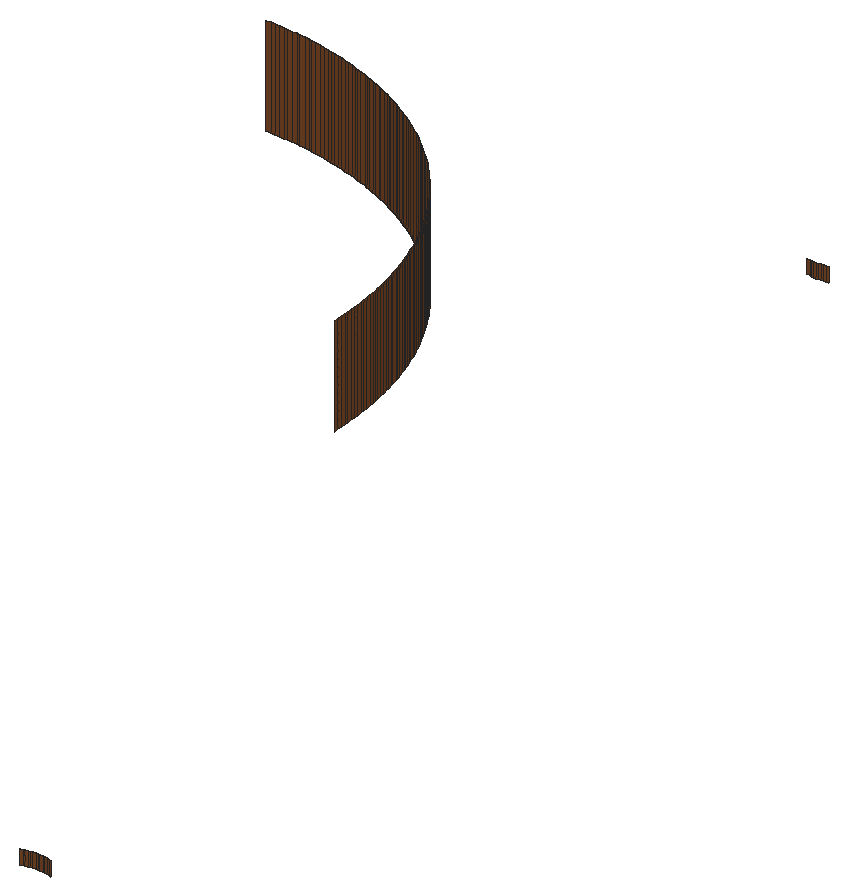
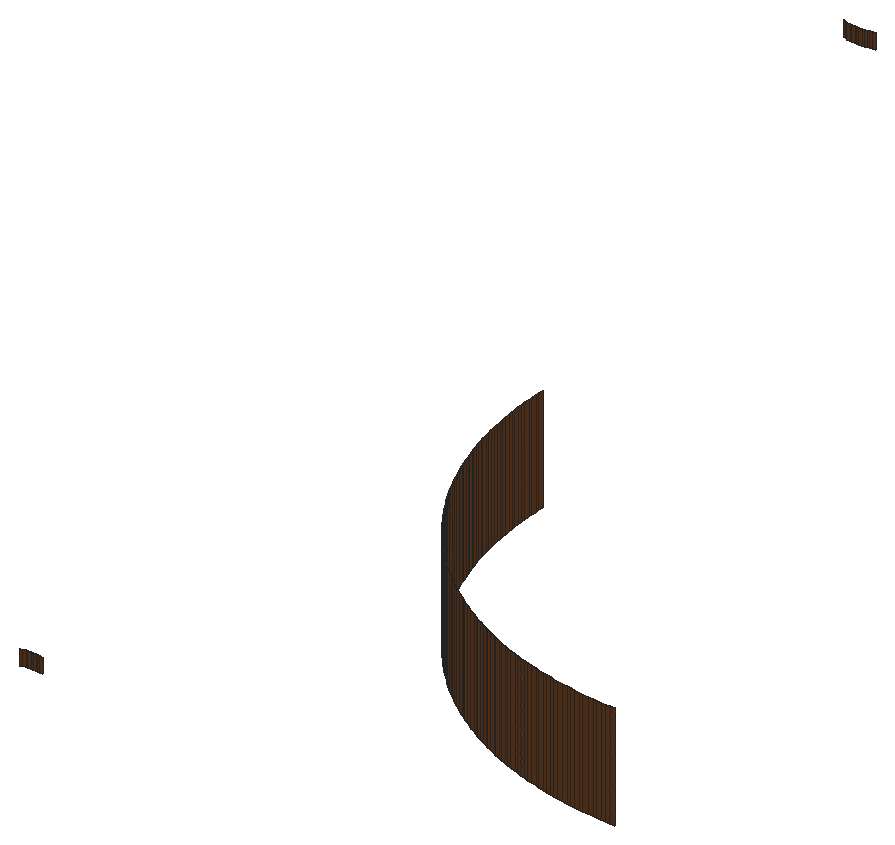
# SketchUp Ruby script. Lengths in inches.
U = 1.inch
M = Sketchup.active_model
def pt(a) = Geom::Point3d.new(a.map { |v| v * U })
def face(e, loops, mat)
  f = e.add_face(loops[0].map { |a| pt(a) })
  loops[1..].each { |l| e.add_face(l.map { |a| pt(a) }).erase! }
  f.material = f.back_material = mat if mat
  f
end
# faces: each face lists its corners as indices into pts; further lists are holes
def faces(e, pts, list, mat = nil) = list.each { |f| face(e, (f[0].is_a?(Array) ? f : [f]).map { |l| l.map { |i| pts[i] } }, mat) }
# xy, xz, yz: faces in a plane at the given z, y or x. An outline is a flat list of corners, or four numbers for a rectangle; further outlines are holes
def ring(l) = l.size == 4 ? [[l[0], l[1]], [l[2], l[1]], [l[2], l[3]], [l[0], l[3]]] : l.each_slice(2).to_a
def flat(e, list, mat, &to3) = list.each { |f| face(e, (f[0].is_a?(Array) ? f : [f]).map { |l| ring(l).map { |u, v| to3.(u, v) } }, mat) }
def xy(e, z, list, mat = nil) = flat(e, list, mat) { |x, y| [x, y, z] }
def xz(e, y, list, mat = nil) = flat(e, list, mat) { |x, z| [x, y, z] }
def yz(e, x, list, mat = nil) = flat(e, list, mat) { |y, z| [x, y, z] }
def lines(e, pts, list) = list.each { |a, b| e.add_line(pt(pts[a]), pt(pts[b])) }
# prism: a flat outline (further loops are holes) pulled along v
def prism(e, loops, v, mat = nil)
  f = face(e, loops, mat); d = Geom::Vector3d.new(v.map { |x| x * U })
  f.pushpull(f.normal.samedirection?(d) ? d.length : -d.length)
end
def box(e, o, s, mat = nil) = prism(e, [[o, [o[0] + s[0], o[1], o[2]], [o[0] + s[0], o[1] + s[1], o[2]], [o[0], o[1] + s[1], o[2]]]], [0, 0, s[2]], mat)
def at(x, y, z, deg = 0) = Geom::Transformation.translation(pt([x, y, z])) * Geom::Transformation.rotation(ORIGIN, Z_AXIS, deg.degrees)
def axes(o, x, y, z) = Geom::Transformation.new([*x, 0, *y, 0, *z, 0, *pt(o).to_a, 1])
def part(name) = M.definitions.add(name)
# library, detail: a bought-in or finely detailed component or shape, given as its bounding box
def library(name, o, s) = part(name).tap { |d| box(d.entities, o, s) }
def detail(e, o, s) = box(e.add_group.entities, o, s)
def put(e, d, t, mat = nil) = e.add_instance(d, t).tap { |i| i.material = mat if mat }
def group(e, t, mat = nil) = e.add_group.tap { |g| g.transformation = t; g.material = mat if mat }.entities
root = M.entities
M.materials.add("[Wood Veneer 01]3").color = [120, 70, 37]
xz(root,128.66,[[147.1,118,147.18,118.5]],"[Wood Veneer 01]3")
xz(root,128.67,[[146.93,118,147.01,118.5]],"[Wood Veneer 01]3")
xz(root,165,[[126,118,126.16,121.5],[126.16,118,126.3125,121.5]],"[Wood Veneer 01]3")
xz(root,168,[[142.9,118,142.99,118.5],[142.99,118,143.07,118.5]],"[Wood Veneer 01]3")
xz(root,168.01,[[143.15,118,143.24,118.5]],"[Wood Veneer 01]3")
yz(root,138,[[153,118,153.16,121.5],[153.16,118,153.3125,121.5]],"[Wood Veneer 01]3")
p = [[146.44,128.59,118],[146.52,128.61,118],[146.52,128.61,118.5],[146.44,128.59,118.5],[146.6,128.625,118],[146.6,128.625,118.5],
  [146.68,128.64,118],[146.68,128.64,118.5],[146.76,128.65,118],[146.76,128.65,118.5],[147.18,128.66,118],[147.26,128.65,118],
  [147.26,128.65,118.5],[147.18,128.66,118.5],[147.35,128.64,118],[147.43,128.62,118],[147.43,128.62,118.5],[147.35,128.64,118.5],
  [147.51,128.6,118],[147.51,128.6,118.5],[146.85,128.66,118],[146.85,128.66,118.5],[146.93,128.67,118],[146.93,128.67,118.5],
  [147.01,128.67,118],[147.1,128.66,118],[147.1,128.66,118.5],[147.01,128.67,118.5],[138,153.3125,118],[138,153.3125,121],
  [138,153.3125,121.5],[137.99,153.47,121.5],[137.99,153.47,121],[137.99,153.47,118],[137.98,153.63,121.5],[137.98,153.63,121],
  [137.98,153.63,118],[137.97,153.78,121.5],[137.97,153.78,121],[137.97,153.78,118],[137.96,153.94,121.5],[137.96,153.94,121],
  [137.96,153.94,118],[137.95,154.1,121.5],[137.95,154.1,121],[137.95,154.1,118],[137.93,154.25,121.5],[137.93,154.25,121],
  [137.93,154.25,118],[137.92,154.41,121.5],[137.92,154.41,121],[137.92,154.41,118],[137.9,154.57,121.5],[137.9,154.57,121],
  [137.9,154.57,118],[137.875,154.72,121.5],[137.875,154.72,121],[137.875,154.72,118],[137.85,154.88,121.5],[137.85,154.88,121],
  [137.85,154.88,118],[137.83,155.03,121.5],[137.83,155.03,121],[137.83,155.03,118],[137.8,155.1875,121.5],[137.8,155.1875,121],
  [137.8,155.1875,118],[137.77,155.34,121.5],[137.77,155.34,121],[137.77,155.34,118],[137.74,155.49,121.5],[137.74,155.49,121],
  [137.74,155.49,118],[137.7,155.65,121.5],[137.7,155.65,121],[137.7,155.65,118],[137.67,155.8,121.5],[137.67,155.8,121],
  [137.67,155.8,118],[137.63,155.95,121.5],[137.63,155.95,121],[137.63,155.95,118],[137.59,156.11,121.5],[137.59,156.11,121],
  [137.59,156.11,118],[137.55,156.26,121.5],[137.55,156.26,121],[137.55,156.26,118],[137.51,156.41,121.5],[137.51,156.41,121],
  [137.51,156.41,118],[137.46,156.56,121.5],[137.46,156.56,121],[137.46,156.56,118],[137.41,156.71,121.5],[137.41,156.71,121],
  [137.41,156.71,118],[137.36,156.86,121.5],[137.36,156.86,121],[137.36,156.86,118],[137.3125,157.01,121.5],[137.3125,157.01,121],
  [137.3125,157.01,118],[137.26,157.15,121.5],[137.26,157.15,121],[137.26,157.15,118],[137.2,157.3,121.5],[137.2,157.3,121],
  [137.2,157.3,118],[137.15,157.45,121.5],[137.15,157.45,121],[137.15,157.45,118],[137.09,157.59,121.5],[137.09,157.59,121],
  [137.09,157.59,118],[137.03,157.74,121.5],[137.03,157.74,121],[137.03,157.74,118],[136.96,157.88,121.5],[136.96,157.88,121],
  [136.96,157.88,118],[136.9,158.02,121.5],[136.9,158.02,121],[136.9,158.02,118],[136.83,158.17,121.5],[136.83,158.17,121],
  [136.83,158.17,118],[136.76,158.31,121.5],[136.76,158.31,121],[136.76,158.31,118],[136.69,158.45,121.5],[136.69,158.45,121],
  [136.69,158.45,118],[136.62,158.59,121.5],[136.62,158.59,121],[136.62,158.59,118],[136.55,158.73,121.5],[136.55,158.73,121],
  [136.55,158.73,118],[136.47,158.86,121.5],[136.47,158.86,121],[136.47,158.86,118],[136.39,159,121.5],[136.39,159,121],
  [136.39,159,118],[136.3125,159.14,121.5],[136.3125,159.14,121],[136.3125,159.14,118],[136.23,159.27,121.5],[136.23,159.27,121],
  [136.23,159.27,118],[136.15,159.4,121.5],[136.15,159.4,121],[136.15,159.4,118],[136.0625,159.54,121.5],[136.0625,159.54,121],
  [136.0625,159.54,118],[135.98,159.67,121.5],[135.98,159.67,121],[135.98,159.67,118],[135.89,159.8,121.5],[135.89,159.8,121],
  [135.89,159.8,118],[135.8,159.93,121.5],[135.8,159.93,121],[135.8,159.93,118],[135.71,160.05,121.5],[135.71,160.05,121],
  [135.71,160.05,118],[135.62,160.18,121.5],[135.62,160.18,121],[135.62,160.18,118],[135.52,160.31,121.5],[135.52,160.31,121],
  [135.52,160.31,118],[135.42,160.43,121.5],[135.42,160.43,121],[135.42,160.43,118],[135.33,160.55,121.5],[135.33,160.55,121],
  [135.33,160.55,118],[135.23,160.67,121.5],[135.23,160.67,121],[135.23,160.67,118],[135.125,160.79,121.5],[135.125,160.79,121],
  [135.125,160.79,118],[135.02,160.91,121.5],[135.02,160.91,121],[135.02,160.91,118],[134.92,161.03,121.5],[134.92,161.03,121],
  [134.92,161.03,118],[134.8125,161.15,121.5],[134.8125,161.15,121],[134.8125,161.15,118],[134.7,161.26,121.5],[134.7,161.26,121],
  [134.7,161.26,118],[134.6,161.375,121.5],[134.6,161.375,121],[134.6,161.375,118],[134.49,161.49,121.5],[134.49,161.49,121],
  [134.49,161.49,118],[134.375,161.6,121.5],[134.375,161.6,121],[134.375,161.6,118],[134.26,161.7,121.5],[134.26,161.7,121],
  [134.26,161.7,118],[134.15,161.8125,121.5],[134.15,161.8125,121],[134.15,161.8125,118],[134.03,161.92,121.5],[134.03,161.92,121],
  [134.03,161.92,118],[133.91,162.02,121.5],[133.91,162.02,121],[133.91,162.02,118],[133.79,162.125,121.5],[133.79,162.125,121],
  [133.79,162.125,118],[133.67,162.23,121.5],[133.67,162.23,121],[133.67,162.23,118],[133.55,162.33,121.5],[133.55,162.33,121],
  [133.55,162.33,118],[133.43,162.42,121.5],[133.43,162.42,121],[133.43,162.42,118],[133.31,162.52,121.5],[133.31,162.52,121],
  [133.31,162.52,118],[133.18,162.62,121.5],[133.18,162.62,121],[133.18,162.62,118],[133.05,162.71,121.5],[133.05,162.71,121],
  [133.05,162.71,118],[132.93,162.8,121.5],[132.93,162.8,121],[132.93,162.8,118],[132.8,162.89,121.5],[132.8,162.89,121],
  [132.8,162.89,118],[132.67,162.98,121.5],[132.67,162.98,121],[132.67,162.98,118],[132.54,163.0625,121.5],[132.54,163.0625,121],
  [132.54,163.0625,118],[132.4,163.15,118],[132.4,163.15,121],[132.4,163.15,121.5],[132.27,163.23,121.5],[132.27,163.23,121],
  [132.27,163.23,118],[132.14,163.3125,121.5],[132.14,163.3125,121],[132.14,163.3125,118],[132,163.39,121.5],[132,163.39,121],
  [132,163.39,118],[131.86,163.47,121.5],[131.86,163.47,121],[131.86,163.47,118],[131.73,163.55,118],[131.73,163.55,121],
  [131.73,163.55,121.5],[131.59,163.62,121.5],[131.59,163.62,121],[131.59,163.62,118],[131.45,163.69,121.5],[131.45,163.69,121],
  [131.45,163.69,118],[131.31,163.76,121.5],[131.31,163.76,121],[131.31,163.76,118],[131.17,163.83,118],[131.17,163.83,121],
  [131.17,163.83,121.5],[131.02,163.9,121.5],[131.02,163.9,121],[131.02,163.9,118],[130.88,163.96,121.5],[130.88,163.96,121],
  [130.88,163.96,118],[130.74,164.03,118],[130.74,164.03,121],[130.74,164.03,121.5],[130.59,164.09,121.5],[130.59,164.09,121],
  [130.59,164.09,118],[130.45,164.15,118],[130.45,164.15,121],[130.45,164.15,121.5],[130.3,164.2,121.5],[130.3,164.2,121],
  [130.3,164.2,118],[130.15,164.26,121.5],[130.15,164.26,121],[130.15,164.26,118],[130.01,164.3125,118],[130.01,164.3125,121],
  [130.01,164.3125,121.5],[129.86,164.36,121.5],[129.86,164.36,121],[129.86,164.36,118],[129.71,164.41,118],[129.71,164.41,121],
  [129.71,164.41,121.5],[129.56,164.46,121.5],[129.56,164.46,121],[129.56,164.46,118],[129.26,164.55,118],[129.26,164.55,121],
  [129.26,164.55,121.5],[129.11,164.59,121.5],[129.11,164.59,121],[129.11,164.59,118],[129.41,164.51,118],[129.41,164.51,121],
  [129.41,164.51,121.5],[128.95,164.63,118],[128.95,164.63,121],[128.95,164.63,121.5],[128.8,164.67,121.5],[128.8,164.67,121],
  [128.8,164.67,118],[128.49,164.74,118],[128.49,164.74,121],[128.49,164.74,121.5],[128.34,164.77,121.5],[128.34,164.77,121],
  [128.34,164.77,118],[128.65,164.7,118],[128.65,164.7,121],[128.65,164.7,121.5],[128.03,164.83,118],[128.03,164.83,121],
  [128.03,164.83,121.5],[127.88,164.85,121.5],[127.88,164.85,121],[127.88,164.85,118],[128.1875,164.8,118],[128.1875,164.8,121],
  [128.1875,164.8,121.5],[127.1,164.95,118],[127.1,164.95,121],[127.1,164.95,121.5],[126.94,164.96,121.5],[126.94,164.96,121],
  [126.94,164.96,118],[127.25,164.93,118],[127.25,164.93,121],[127.25,164.93,121.5],[127.41,164.92,118],[127.41,164.92,121],
  [127.41,164.92,121.5],[127.57,164.9,118],[127.57,164.9,121],[127.57,164.9,121.5],[127.72,164.875,118],[127.72,164.875,121],
  [127.72,164.875,121.5],[126.47,164.99,118],[126.47,164.99,121],[126.47,164.99,121.5],[126.3125,165,121.5],[126.3125,165,121],
  [126.3125,165,118],[126.63,164.98,118],[126.63,164.98,121],[126.63,164.98,121.5],[126.78,164.97,118],[126.78,164.97,121],
  [126.78,164.97,121.5],[142.82,168.01,118],[142.74,168.02,118],[142.74,168.02,118.5],[142.82,168.01,118.5],[142.65,168.03,118],
  [142.65,168.03,118.5],[142.9,168,118],[142.9,168,118.5],[143.15,168.01,118],[143.07,168,118],[143.07,168,118.5],
  [143.15,168.01,118.5],[143.32,168.03,118],[143.24,168.01,118],[143.24,168.01,118.5],[143.32,168.03,118.5],[143.4,168.04,118],
  [143.4,168.04,118.5]]
faces(root,p,[[0,1,2,3],[1,4,5,2],[4,6,7,5],[6,8,9,7],[10,11,12,13],[14,15,16,17],[11,14,17,12],[15,18,19,16],
  [8,20,21,9],[20,22,23,21],[24,25,26,27],[28,29,30,31,32,33],[33,32,31,34,35,36],[36,35,34,37,38,39],[39,38,37,40,41,42],[42,41,40,43,44,45],
  [45,44,43,46,47,48],[48,47,46,49,50,51],[51,50,49,52,53,54],[54,53,52,55,56,57],[57,56,55,58,59,60],[60,59,58,61,62,63],[63,62,61,64,65,66],[66,65,64,67,68,69],
  [69,68,67,70,71,72],[72,71,70,73,74,75],[75,74,73,76,77,78],[78,77,76,79,80,81],[81,80,79,82,83,84],[84,83,82,85,86,87],[87,86,85,88,89,90],[90,89,88,91,92,93],
  [93,92,91,94,95,96],[96,95,94,97,98,99],[99,98,97,100,101,102],[102,101,100,103,104,105],[105,104,103,106,107,108],[108,107,106,109,110,111],[111,110,109,112,113,114],[114,113,112,115,116,117],
  [117,116,115,118,119,120],[120,119,118,121,122,123],[123,122,121,124,125,126],[126,125,124,127,128,129],[129,128,127,130,131,132],[132,131,130,133,134,135],[135,134,133,136,137,138],[138,137,136,139,140,141],
  [141,140,139,142,143,144],[144,143,142,145,146,147],[147,146,145,148,149,150],[150,149,148,151,152,153],[153,152,151,154,155,156],[156,155,154,157,158,159],[159,158,157,160,161,162],[162,161,160,163,164,165],
  [165,164,163,166,167,168],[168,167,166,169,170,171],[171,170,169,172,173,174],[174,173,172,175,176,177],[177,176,175,178,179,180],[180,179,178,181,182,183],[183,182,181,184,185,186],[186,185,184,187,188,189],
  [189,188,187,190,191,192],[192,191,190,193,194,195],[195,194,193,196,197,198],[198,197,196,199,200,201],[201,200,199,202,203,204],[204,203,202,205,206,207],[207,206,205,208,209,210],[210,209,208,211,212,213],
  [213,212,211,214,215,216],[216,215,214,217,218,219],[219,218,217,220,221,222],[222,221,220,223,224,225],[225,224,223,226,227,228],[228,227,226,229,230,231],[231,230,229,232,233,234],[234,233,232,235,236,237],
  [237,236,235,238,239,240],[240,239,238,241,242,243],[243,242,241,244,245,246],[246,245,244,247,248,249],[249,248,247,250,251,252],[253,254,255,256,257,258],[252,251,250,255,254,253],[258,257,256,259,260,261],
  [261,260,259,262,263,264],[264,263,262,265,266,267],[268,269,270,271,272,273],[267,266,265,270,269,268],[273,272,271,274,275,276],[276,275,274,277,278,279],[280,281,282,283,284,285],[279,278,277,282,281,280],
  [285,284,283,286,287,288],[289,290,291,292,293,294],[288,287,286,291,290,289],[295,296,297,298,299,300],[294,293,292,297,296,295],[300,299,298,301,302,303],[304,305,306,307,308,309],[303,302,301,306,305,304],
  [310,311,312,313,314,315],[309,308,307,312,311,310],[316,317,318,319,320,321],[322,323,324,318,317,316],[315,314,313,324,323,322],[325,326,327,328,329,330],[321,320,319,327,326,325],[331,332,333,334,335,336],
  [337,338,339,333,332,331],[330,329,328,339,338,337],[340,341,342,343,344,345],[346,347,348,342,341,340],[336,335,334,348,347,346],[349,350,351,352,353,354],[355,356,357,351,350,349],[358,359,360,357,356,355],
  [361,362,363,360,359,358],[364,365,366,363,362,361],[345,344,343,366,365,364],[367,368,369,370,371,372],[373,374,375,369,368,367],[376,377,378,375,374,373],[354,353,352,378,377,376],[379,380,381,382],
  [380,383,384,381],[385,379,382,386],[387,388,389,390],[391,392,393,394],[395,391,394,396]],"[Wood Veneer 01]3")
